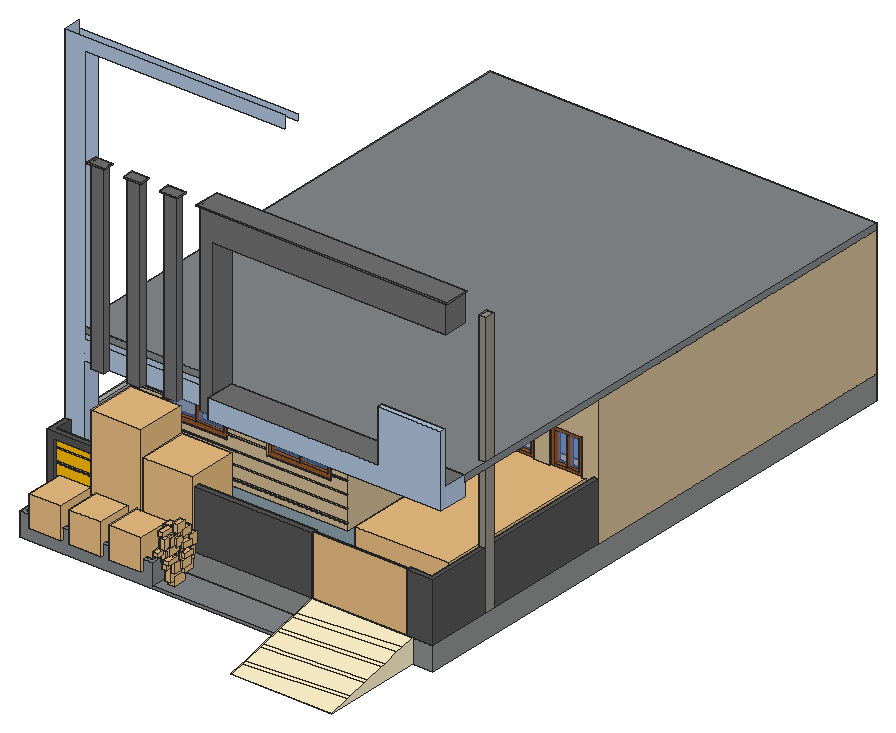
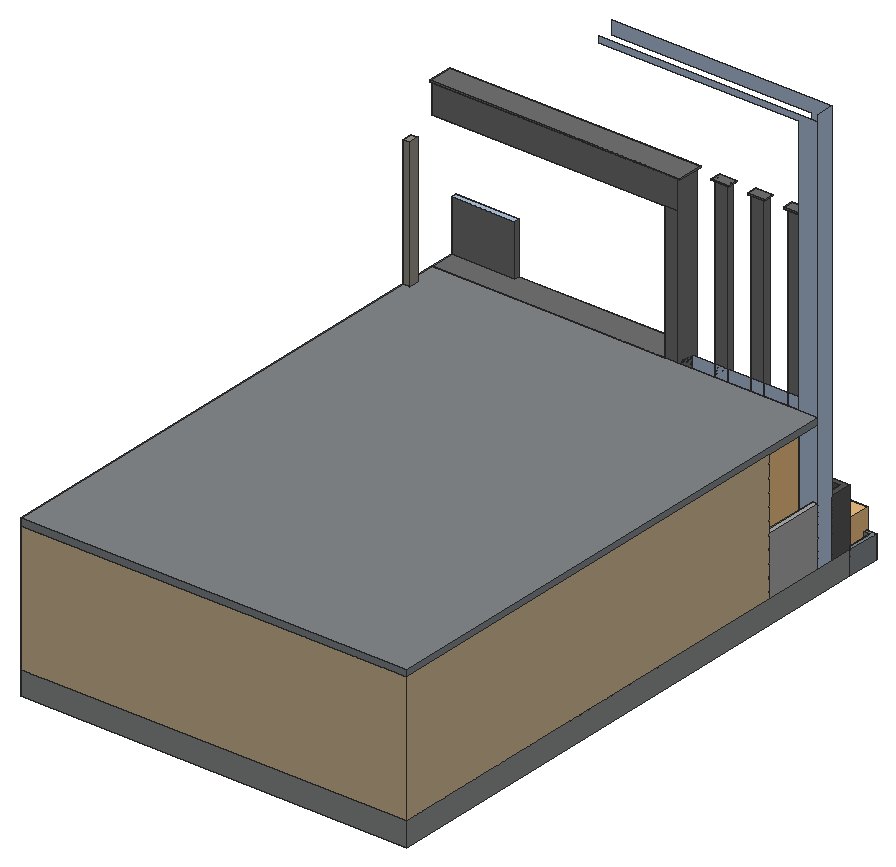
# SketchUp Ruby script. Lengths in inches.
U = 1.inch
M = Sketchup.active_model
def pt(a) = Geom::Point3d.new(a.map { |v| v * U })
def face(e, loops, mat)
  f = e.add_face(loops[0].map { |a| pt(a) })
  loops[1..].each { |l| e.add_face(l.map { |a| pt(a) }).erase! }
  f.material = f.back_material = mat if mat
  f
end
# faces: each face lists its corners as indices into pts; further lists are holes
def faces(e, pts, list, mat = nil) = list.each { |f| face(e, (f[0].is_a?(Array) ? f : [f]).map { |l| l.map { |i| pts[i] } }, mat) }
# xy, xz, yz: faces in a plane at the given z, y or x. An outline is a flat list of corners, or four numbers for a rectangle; further outlines are holes
def ring(l) = l.size == 4 ? [[l[0], l[1]], [l[2], l[1]], [l[2], l[3]], [l[0], l[3]]] : l.each_slice(2).to_a
def flat(e, list, mat, &to3) = list.each { |f| face(e, (f[0].is_a?(Array) ? f : [f]).map { |l| ring(l).map { |u, v| to3.(u, v) } }, mat) }
def xy(e, z, list, mat = nil) = flat(e, list, mat) { |x, y| [x, y, z] }
def xz(e, y, list, mat = nil) = flat(e, list, mat) { |x, z| [x, y, z] }
def yz(e, x, list, mat = nil) = flat(e, list, mat) { |y, z| [x, y, z] }
def lines(e, pts, list) = list.each { |a, b| e.add_line(pt(pts[a]), pt(pts[b])) }
# prism: a flat outline (further loops are holes) pulled along v
def prism(e, loops, v, mat = nil)
  f = face(e, loops, mat); d = Geom::Vector3d.new(v.map { |x| x * U })
  f.pushpull(f.normal.samedirection?(d) ? d.length : -d.length)
end
def box(e, o, s, mat = nil) = prism(e, [[o, [o[0] + s[0], o[1], o[2]], [o[0] + s[0], o[1] + s[1], o[2]], [o[0], o[1] + s[1], o[2]]]], [0, 0, s[2]], mat)
def at(x, y, z, deg = 0) = Geom::Transformation.translation(pt([x, y, z])) * Geom::Transformation.rotation(ORIGIN, Z_AXIS, deg.degrees)
def axes(o, x, y, z) = Geom::Transformation.new([*x, 0, *y, 0, *z, 0, *pt(o).to_a, 1])
def part(name) = M.definitions.add(name)
# library, detail: a bought-in or finely detailed component or shape, given as its bounding box
def library(name, o, s) = part(name).tap { |d| box(d.entities, o, s) }
def detail(e, o, s) = box(e.add_group.entities, o, s)
def put(e, d, t, mat = nil) = e.add_instance(d, t).tap { |i| i.material = mat if mat }
def group(e, t, mat = nil) = e.add_group.tap { |g| g.transformation = t; g.material = mat if mat }.entities
root = M.entities
M.materials.add("[0099_LightSteelBlue]").color = [176, 196, 222]
M.materials.add("[Blacktop Old 01]").color = [132, 136, 139]
M.materials.add("[Blacktop Old 02]").color = [143, 145, 145]
M.materials.add("[Color D01]").color = [255, 242, 204]
M.materials.add("[Color D04]").color = [255, 204, 50]
M.materials.add("[Color D05]").color = [255, 191, 0]
M.materials.add("[Color M03]").color = [170, 170, 170]
M.materials.add("[Color M05]").color = [114, 114, 114]
M.materials.add("[Color M06]").color = [86, 86, 86]
M.materials.add("[Formica Beige]").color = [211, 187, 149]
M.materials.add("[Formica Graystone]").color = [149, 146, 135]
M.materials.add("[Square Glass Tile 01]").color = [123, 142, 151]
M.materials.add("[Translucent Glass Blue]").color = [100, 149, 237]
M.materials["[Translucent Glass Blue]"].alpha = 0.5
M.materials.add("[Wood Cherry Original]").color = [152, 86, 42]
c1 = library("Group59\#1",[-32.98,33.92,22.15],[23.96,96.56,83.1])
c2 = library("Group60\#1",[-47.26,-81.53,115.8],[11.57,60.71,53.88])
c3 = library("Group61\#1",[17.15,84.19,16.4],[76.98,72.79,100.38])
c4 = library("Group62\#1",[-41.8,-20.16,82.85],[99.48,139.14,54.12])
c5 = library("Group63\#1",[-78.07,100.88,62.43],[61.26,81.43,86.37])
c6 = library("Group64\#1",[46.33,-12.9,51.95],[92.42,78.95,51.57])
c7 = library("Group65\#1",[-73.78,-20.03,120.09],[33.05,103.71,51.96])
c8 = library("Group66\#1",[-93.39,-19.9375,115.15],[70.74,15.37,89.07])
c9 = library("Group67\#1",[-160.6,-41.84,176.32],[92.55,73.84,45.89])
c10 = library("Group68\#1",[-72.58,-136.32,72.38],[80.41,85.97,95.72])
c11 = library("Group69\#1",[-107.89,47.83,91.71],[66.48,87.86,82.46])
c12 = library("Group70\#1",[-20.98,-42.53,-198.63],[46.69,46.24,172.61])
c13 = library("Group71\#1",[-0.8,-43.35,191.05],[81.04,80.57,74.82])
c14 = library("Group72\#1",[-44.16,-20.64,117.23],[64.94,35.73,104.26])
c15 = library("Group73\#2",[-85.2,-151.09,191.26],[83.6,108.34,38.47])
c16 = library("Group74\#1",[-43.32,-82.39,113.66],[8.74,67.58,95.91])
c17 = library("Group75\#1",[-19.52,-83.01,-122.96],[25.03,96.75,107.02])
c18 = library("Group76\#1",[-73.41,104.74,-36.57],[91.05,64.11,87.76])
c19 = library("Group77\#1",[6.72,-35.5625,-44.3],[97.86,50.43,71.28])
c20 = library("Group78\#1",[-46.16,95.67,-127.18],[89.22,60,98.58])
c21 = library("Group79\#1",[-73.36,-53.98,-265.87],[113.5,113.5,80.32])
c22 = library("Group80\#1",[-49.58,-31.64,-192.73],[34.2,35.75,335.89])
c23 = library("Group81\#1",[-33.25,31.15,20.5625],[19.21,100.94,38.88])
c24 = library("Group82\#1",[70.71,-26.24,-13.72],[94.01,86.31,40.81])
c25 = library("Group83\#1",[-78.76,-45.9375,-42.49],[89.36,13.07,73.45])
c26 = library("Group84\#1",[1.95,9.69,-124.66],[99.34,14.87,96.07])
c27 = library("Group85\#1",[5.34,-106.29,-47.41],[68.63,73.37,61.51])
c28 = library("Group86\#1",[4.23,10.03,-136.62],[40.98,41.87,51.36])
c29 = library("Group87\#1",[7.14,-44.59,-77.7],[48.84,15.98,59.8])
c30 = library("Group88\#1",[-32.7,-24.31,24.45],[55.13,61.32,79.5])
c31 = library("Group89\#1",[-77.24,-123.58,-46.56],[87.79,92.59,104.1])
c32 = library("Group90\#1",[-164.72,37.75,-20.84],[98.29,65.97,82.77])
c33 = library("Group91\#1",[-103.43,33.69,20.61],[71.41,32.36,40.62])
c34 = library("Group92\#1",[-125.68,-182.3125,23.5],[85.66,94.28,35.8])
c35 = library("Group93\#1",[5.2,-33.94,-67.23],[20.18,157.98,40.35])
c36 = library("Group94\#1",[2.39,9.02,-121.59],[42.15,71.34,93.56])
c37 = library("Group95\#1",[-55.3125,-129.29,-96.66],[79.37,72.9,68.93])
c38 = library("Group96\#1",[-140.7,-35.21,-77.44],[97.31,70.81,56.29])
c39 = library("Group97\#1",[-10.06,-56.42,72.68],[90.9,68.8,76.87])
c40 = library("Group98\#1",[12.8,58.29,-66.98],[80.58,78.21,79.14])
c41 = library("Group99\#1",[-35.4,-17.16,23.02],[118.23,50.83,58.94])
c42 = library("Group100\#1",[29.51,-171.04,-20.53],[91.11,101.22,39.04])
c43 = library("Group101\#1",[-97.95,11.13,-121.05],[102.09,51.91,53.69])
c44 = library("Group102\#1",[6.02,5.95,144.49],[89.45,87.47,55.68])
c45 = library("Group103\#1",[-45.73,-21.24,120.09],[87.14,68.72,79.33])
c46 = library("Group104\#1",[-32.38,-52.6,16.55],[60.96,98.07,53.51])
c47 = library("Group105\#1",[-69.28,-88.77,-223.3],[101.83,125.23,376.24])
c48 = library("Group106\#1",[-122.02,-42.04,23.03],[89.8,79.69,89.2])
c49 = library("Group107\#1",[-147.28,-98.05,24.68],[53.49,99.81,98.14])
c50 = library("Group108\#1",[38.95,-94,-129.36],[60.91,93.27,90.52])
c51 = library("Group109\#1",[-124.75,-75.19,-35.84],[77.11,72.51,79.94])
c52 = library("Group110\#1",[-78.58,0.56,-119.09],[84.31,12.02,77.58])
c53 = library("Group111\#1",[62.69,-31.6,-103.24],[86.45,84.15,71.79])
c54 = library("Group112\#1",[5.13,22.77,-174.65],[91.17,82.67,75.7])
c55 = library("Group113\#1",[-8.89,-115.37,23.85],[66.54,93.07,62.51])
c56 = library("Group114\#1",[-138.5625,33.88,-184.78],[81.4,51.14,109.21])
c57 = library("Group115\#1",[-39.22,1.8,-197.74],[25.16,42.04,242.32])
c58 = library("Group116\#1",[-16.77,0.31,-197.58],[31.04,19.97,97.43])
c59 = part("Group58\#1")
put(c59.entities,c1,at(0,0,0))
put(c59.entities,c2,at(0,0,0))
put(c59.entities,c3,at(0,0,0))
put(c59.entities,c4,at(0,0,0))
put(c59.entities,c5,at(0,0,0))
put(c59.entities,c6,at(0,0,0))
put(c59.entities,c7,at(0,0,0))
put(c59.entities,c8,at(0,0,0))
put(c59.entities,c9,at(0,0,0))
put(c59.entities,c10,at(0,0,0))
put(c59.entities,c11,at(0,0,0))
put(c59.entities,c12,at(0,0,0))
put(c59.entities,c13,at(0,0,0))
put(c59.entities,c14,at(0,0,0))
put(c59.entities,c15,at(0,0,0))
put(c59.entities,c16,at(0,0,0))
put(c59.entities,c17,at(0,0,0))
put(c59.entities,c18,at(0,0,0))
put(c59.entities,c19,at(0,0,0))
put(c59.entities,c20,at(0,0,0))
put(c59.entities,c21,at(0,0,0))
put(c59.entities,c22,at(0,0,0))
put(c59.entities,c23,at(0,0,0))
put(c59.entities,c24,at(0,0,0))
put(c59.entities,c25,at(0,0,0))
put(c59.entities,c26,at(0,0,0))
put(c59.entities,c27,at(0,0,0))
put(c59.entities,c28,at(0,0,0))
put(c59.entities,c29,at(0,0,0))
put(c59.entities,c30,at(0,0,0))
put(c59.entities,c31,at(0,0,0))
put(c59.entities,c32,at(0,0,0))
put(c59.entities,c33,at(0,0,0))
put(c59.entities,c34,at(0,0,0))
put(c59.entities,c35,at(0,0,0))
put(c59.entities,c36,at(0,0,0))
put(c59.entities,c37,at(0,0,0))
put(c59.entities,c38,at(0,0,0))
put(c59.entities,c39,at(0,0,0))
put(c59.entities,c40,at(0,0,0))
put(c59.entities,c41,at(0,0,0))
put(c59.entities,c42,at(0,0,0))
put(c59.entities,c43,at(0,0,0))
put(c59.entities,c44,at(0,0,0))
put(c59.entities,c45,at(0,0,0))
put(c59.entities,c46,at(0,0,0))
put(c59.entities,c47,at(0,0,0))
put(c59.entities,c48,at(0,0,0))
put(c59.entities,c49,at(0,0,0))
put(c59.entities,c50,at(0,0,0))
put(c59.entities,c51,at(0,0,0))
put(c59.entities,c52,at(0,0,0))
put(c59.entities,c53,at(0,0,0))
put(c59.entities,c54,at(0,0,0))
put(c59.entities,c55,at(0,0,0))
put(c59.entities,c56,at(0,0,0))
put(c59.entities,c57,at(0,0,0))
put(c59.entities,c58,at(0,0,0))
c60 = part("SimLab\#1")
put(c60.entities,c59,at(0,0,0))
c61 = library("mercy",[0,0.0625,0.17],[86.93,197.26,61.05])
c62 = library("SKT_Nearly Natural 5' Kentia Palm Silk Tree",[-23.18,-17.61,0],[47.48,43.95,59.125])
c63 = library("Untitled",[0,0,0],[36,4.39,84])
c64 = part("Group48\#1")
prism(c64.entities,[[[1382.99,-93.96,0],[1358.12,-93.96,0],[1358.12,-88.96,0],[1377.99,-88.96,0],[1377.99,98,0],[1382.99,98,0]]],[0,0,54.37])
c65 = part("Group50\#1")
box(c65.entities,[1024.5625,-57.52,0],[5,57.52,54.37])
c66 = part("Group51\#1")
xy(c66.entities,0,[[1024.5625,-93.96,1024.5625,-72.96,1029.5625,-72.96,1029.5625,-88.96,1270.5,-88.96,1270.5,-93.96,1136.9375,-93.96,1136.9375,-90.96,1030.5625,-90.96,1030.5625,-93.96]])
xy(c66.entities,3.55,[[1030.5625,-90.96,1136.9375,-89.96]])
xy(c66.entities,5.49,[[1030.5625,-90.96,1136.9375,-89.96]])
xy(c66.entities,15.37,[[1030.5625,-90.96,1136.9375,-89.96]])
xy(c66.entities,17.3,[[1030.5625,-90.96,1136.9375,-89.96]])
xy(c66.entities,27.18,[[1030.5625,-90.96,1136.9375,-89.96]])
xy(c66.entities,29.12,[[1030.5625,-90.96,1136.9375,-89.96]])
xy(c66.entities,38.99,[[1030.5625,-90.96,1136.9375,-89.96]])
xy(c66.entities,40.93,[[1030.5625,-90.96,1136.9375,-89.96]])
xy(c66.entities,48.37,[[1030.5625,-93.96,1136.9375,-90.96]])
xy(c66.entities,54.37,[[1024.5625,-93.96,1270.5,-93.96,1270.5,-88.96,1029.5625,-88.96,1029.5625,-72.96,1024.5625,-72.96]])
xz(c66.entities,-93.96,[[1024.5625,0,1030.5625,0,1030.5625,48.37,1136.9375,48.37,1136.9375,0,1270.5,0,1270.5,54.37,1024.5625,54.37]])
xz(c66.entities,-90.96,[[1030.5625,0,1136.9375,3.55]])
xz(c66.entities,-90.96,[[1030.5625,5.49,1136.9375,15.37],[1030.5625,17.3,1136.9375,27.18],[1030.5625,29.12,1136.9375,38.99],[1030.5625,40.93,1136.9375,48.37]],"[Color D05]")
xz(c66.entities,-89.96,[[1030.5625,3.55,1136.9375,5.49],[1030.5625,15.37,1136.9375,17.3]],"[Color D04]")
xz(c66.entities,-89.96,[[1030.5625,27.18,1136.9375,29.12],[1030.5625,38.99,1136.9375,40.93]],"[Color D05]")
xz(c66.entities,-88.96,[[1029.5625,0,1270.5,54.37]])
xz(c66.entities,-72.96,[[1024.5625,0,1029.5625,54.37]])
yz(c66.entities,1024.5625,[[-93.96,0,-72.96,54.37]])
yz(c66.entities,1029.5625,[[-88.96,0,-72.96,54.37]])
yz(c66.entities,1030.5625,[[-93.96,0,-90.96,48.37]])
yz(c66.entities,1136.9375,[[-93.96,0,-90.96,48.37]])
yz(c66.entities,1270.5,[[-93.96,0,-88.96,54.37]])
c67 = library("Untitled\#1",[131.66,19.68,0],[2.41,197.25,46.46])
c68 = part("Group4\#2")
xy(c68.entities,0,[[-26.0625,-20.0625,-0.59,20.0625],[0.59,-20.0625,26.0625,20.0625]])
c69 = part("Group3\#1")
prism(c69.entities,[[[-30,-24,0],[-30,24,0],[30,24,0],[30,-24,0]],[[26.0625,-20.0625,0],[26.0625,20.0625,0],[0.59,20.0625,0],[0.59,-20.0625,0]],[[-0.59,-20.0625,0],[-0.59,20.0625,0],[-26.0625,20.0625,0],[-26.0625,-20.0625,0]]],[0,0,5.875])
put(c69.entities,c68,at(0,0,2.9375),"[Translucent Glass Blue]")
c70 = part("Group6\#2")
xy(c70.entities,0,[[-26.0625,-20.0625,-0.59,20.0625],[0.59,-20.0625,26.0625,20.0625]])
c71 = part("Group5\#1")
prism(c71.entities,[[[-30,-24,0],[-30,24,0],[30,24,0],[30,-24,0]],[[0.59,20.0625,0],[0.59,-20.0625,0],[26.0625,-20.0625,0],[26.0625,20.0625,0]],[[-26.0625,-20.0625,0],[-0.59,-20.0625,0],[-0.59,20.0625,0],[-26.0625,20.0625,0]]],[0,0,5.875])
put(c71.entities,c70,at(0,0,2.9375),"[Translucent Glass Blue]")
c72 = part("Group8\#2")
xy(c72.entities,0,[[-11.0625,-14.0625,-0.59,14.0625],[0.59,-14.0625,11.0625,14.0625]])
c73 = part("Group7\#1")
prism(c73.entities,[[[-15,18,0],[15,18,0],[15,-18,0],[-15,-18,0]],[[11.0625,-14.0625,0],[11.0625,14.0625,0],[0.59,14.0625,0],[0.59,-14.0625,0]],[[-11.0625,-14.0625,0],[-0.59,-14.0625,0],[-0.59,14.0625,0],[-11.0625,14.0625,0]]],[0,0,5.875])
put(c73.entities,c72,at(0,0,2.9375),"[Translucent Glass Blue]")
c74 = part("Group10\#2")
xy(c74.entities,0,[[-10.5625,-14.0625,-0.59,14.0625],[0.59,-14.0625,10.5625,14.0625]])
c75 = part("Group9\#1")
prism(c75.entities,[[[14.5,18,0],[14.5,-18,0],[-14.5,-18,0],[-14.5,18,0]],[[0.59,-14.0625,0],[10.5625,-14.0625,0],[10.5625,14.0625,0],[0.59,14.0625,0]],[[-0.59,-14.0625,0],[-0.59,14.0625,0],[-10.5625,14.0625,0],[-10.5625,-14.0625,0]]],[0,0,5.875])
put(c75.entities,c74,at(0,0,2.9375),"[Translucent Glass Blue]")
xy(root,-21.875,[[245.9375,0,339.4375,93.625]],"[Color D01]")
xy(root,0,[[0,114.625,18,130.0625]],"[0099_LightSteelBlue]")
xy(root,108,[[18,114.625,130.05,130.0625]],"[0099_LightSteelBlue]")
xz(root,93.625,[[245.9375,-21.875,336.625,0],[336.625,-21.875,339.4375,0]])
xz(root,114.625,[[0,0,18,0,18,108,39.93,108,39.93,126,18,126,18,366,203.78,366,203.78,378,0,378],[39.93,108,130.05,126]],"[0099_LightSteelBlue]")
xz(root,130.0625,[[0,0,0,372,203.78,372,203.78,366,18,366,18,126,130.05,126,130.05,108,18,108,18,0]],"[0099_LightSteelBlue]")
yz(root,0,[[114.625,0,130.0625,378]],"[0099_LightSteelBlue]")
yz(root,18,[[114.625,0,130.0625,108]],"[0099_LightSteelBlue]")
yz(root,130.05,[[114.625,108,130.0625,126]],"[0099_LightSteelBlue]")
yz(root,245.9375,[[0,-21.875,12.76,-18.89,16.48,-18.03,32.95,-14.18,36.67,-13.31,52.92,-9.51,56.63,-8.64,70.5,-5.4,75.68,-4.19,93.625,0,93.625,-21.875]],"[Color D01]")
yz(root,339.4375,[[0,-21.875,93.625,-21.875,93.625,0,81.67,-2.79,75.68,-4.19,61.8,-7.43,58.09,-8.3,41.84,-12.1,38.13,-12.97,21.65,-16.82,17.94,-17.68]],"[Color D01]")
p = [[339.4375,0,-21.875],[339.4375,17.94,-17.68],[245.9375,12.76,-18.89],[245.9375,0,-21.875],[245.9375,16.48,-18.03],[339.4375,21.65,-16.82],
  [245.9375,32.95,-14.18],[339.4375,38.13,-12.97],[245.9375,36.67,-13.31],[339.4375,41.84,-12.1],[245.9375,52.92,-9.51],[339.4375,58.09,-8.3],
  [245.9375,56.63,-8.64],[339.4375,61.8,-7.43],[245.9375,70.5,-5.4],[339.4375,75.68,-4.19],[245.9375,75.68,-4.19],[339.4375,81.67,-2.79],
  [245.9375,93.625,0],[339.4375,93.625,0],[336.625,93.625,0],[31.9375,192.08,36],[31.9375,192.08,84],[91.9375,192.08,84],
  [91.9375,192.08,36],[128.47,192.08,36],[128.47,192.08,84],[188.47,192.08,84],[188.47,192.08,36],[269.16,290.08,48],
  [269.16,290.08,84],[298.16,290.08,84],[298.16,290.08,48],[312.74,290.08,48],[312.74,290.08,84],[342.74,290.08,84],
  [342.74,290.08,48],[245.9375,93.625,3.6875],[0,93.625,-21.875],[0,93.625,3.6875],[18,130.0625,114],[18,130.0625,108],
  [18,114.625,114]]
faces(root,p,[[0,1,2,3],[4,2,1,5],[6,4,5,7],[8,6,7,9],[10,8,9,11],[12,10,11,13],[14,12,13,15],[16,14,15,17],
  [18,16,17,19,20]],"[Color D01]")
lines(root,p,[[21,22],[22,23],[23,24],[24,21],[25,26],[26,27],[27,28],[28,25],[29,30],[30,31],[31,32],[32,29],
  [33,34],[34,35],[35,36],[36,33],[18,37],[38,39],[40,41],[42,40]])
g1 = group(root,at(0,187.58,-6),"[Square Glass Tile 01]")
xy(g1,-15.875,[[0,-93.96,358.43,420]],"[Blacktop Old 02]")
xy(g1,6,[[0,-93.96,358.43,420]])
xz(g1,-93.96,[[0,-15.875,358.43,6]],"[Blacktop Old 02]")
xz(g1,420,[[0,-15.875,358.43,6]],"[Blacktop Old 02]")
yz(g1,0,[[-93.96,-15.875,420,6]],"[Blacktop Old 02]")
yz(g1,358.43,[[-93.96,-15.875,420,6]],"[Blacktop Old 02]")
g2 = group(root,at(0,62.69,-21.875),"[Blacktop Old 01]")
xy(g2,0,[[0,0,245.9375,30.93]])
xy(g2,2.24,[[122.97,0,245.9375,30.93]])
xy(g2,11.3,[[3.35,3.35,119.62,27.59]])
xy(g2,21.875,[[[0,0,122.97,30.93],[3.35,3.35,119.62,27.59]]])
xz(g2,0,[[0,0,245.9375,0,245.9375,2.24,122.97,2.24,122.97,21.875,0,21.875]])
xz(g2,3.35,[[3.35,11.3,119.62,21.875]])
xz(g2,27.59,[[3.35,11.3,119.62,21.875]])
xz(g2,30.93,[[0,0,0,21.875,122.97,21.875,122.97,2.24,245.9375,2.24,245.9375,0]])
yz(g2,0,[[0,0,30.93,21.875]])
yz(g2,3.35,[[3.35,11.3,27.59,21.875]])
yz(g2,119.62,[[3.35,11.3,27.59,21.875]])
yz(g2,122.97,[[0,2.24,30.93,21.875]])
yz(g2,245.9375,[[0,0,30.93,2.24]])
put(root,c60,axes([135.92,74.36,8.74],[0.05714,0,0],[0,0.10569,0],[0,0,0.09711]))
put(root,c61,axes([259.47,126.22,-11.25],[1,0,0],[0,0.904,0],[0,0,1]))
put(root,c62,axes([23.92,79.35,-10.58],[0.62565,0,0],[0,1.04371,0],[0,0,0.48546]))
put(root,c62,axes([61.18,79.35,-10.58],[0.62565,0,0],[0,1.04371,0],[0,0,0.48546]))
put(root,c62,axes([98.45,79.35,-10.58],[0.62565,0,0],[0,1.04371,0],[0,0,0.48546]))
put(root,c62,axes([112.3,110.83,-1.16],[0.97,0,0],[0,1.04371,0],[0,0,1.0788]))
put(root,c62,axes([64.43,110.83,-1.16],[0.97,0,0],[0,1.04371,0],[0,0,1.45784]))
put(root,c63,at(217.22,287.67,0))
g3 = group(root,at(0,187.58,0),"[Formica Beige]")
xy(g3,0,[[0,0,0,420,358.43,420,358.43,98,253.22,98,253.22,107,349.43,107,349.43,411,9,411,9,9,194.78,9,194.78,107,217.22,107,217.22,98,203.78,98,203.78,0]])
xy(g3,5.19,[[0,0,203.78,1]])
xy(g3,7.12,[[0,0,203.78,1]])
xy(g3,17,[[0,0,203.78,1]])
xy(g3,18.94,[[0,0,203.78,1]])
xy(g3,28.81,[[0,0,203.78,1]])
xy(g3,30.75,[[0,0,203.78,1]])
xy(g3,36,[[31.9375,0,91.9375,9],[128.47,0,188.47,9]])
xy(g3,40.62,[[0,0,31.9375,1],[91.9375,0,128.47,1],[188.47,0,203.78,1]])
xy(g3,42.56,[[0,0,31.9375,1],[91.9375,0,128.47,1],[188.47,0,203.78,1]])
xy(g3,48,[[269.16,98,298.16,107],[312.74,98,342.74,107]])
xy(g3,52.44,[[0,0,31.9375,1],[91.9375,0,128.47,1],[188.47,0,203.78,1]])
xy(g3,54.37,[[0,0,31.9375,1],[91.9375,0,128.47,1],[188.47,0,203.78,1]])
xy(g3,64.25,[[0,0,31.9375,1],[91.9375,0,128.47,1],[188.47,0,203.78,1]])
xy(g3,66.19,[[0,0,31.9375,1],[91.9375,0,128.47,1],[188.47,0,203.78,1]])
xy(g3,76.06,[[0,0,31.9375,1],[91.9375,0,128.47,1],[188.47,0,203.78,1]])
xy(g3,78,[[0,0,31.9375,1],[91.9375,0,128.47,1],[188.47,0,203.78,1]])
xy(g3,84,[[31.9375,0,91.9375,9],[128.47,0,188.47,9],[217.22,98,253.22,107],[269.16,98,298.16,107],[312.74,98,342.74,107]])
xy(g3,87.87,[[0,0,203.78,1]])
xy(g3,89.81,[[0,0,203.78,1]])
xy(g3,99.69,[[0,0,203.78,1]])
xy(g3,101.62,[[0,0,203.78,1]])
xy(g3,111.5,[[0,0,203.78,1]])
xy(g3,113.44,[[0,0,203.78,1]])
xy(g3,120,[[[0,0,203.78,0,203.78,98,358.43,98,358.43,420,0,420],[9,9,9,411,349.43,411,349.43,107,194.78,107,194.78,9]]])
xz(g3,0,[[0,0,203.78,5.19],[0,7.12,203.78,17],[0,18.94,203.78,28.81],[0,30.75,203.78,30.75,203.78,40.62,188.47,40.62,188.47,36,128.47,36,128.47,40.62,91.9375,40.62,91.9375,36,31.9375,36,31.9375,40.62,0,40.62],[0,42.56,31.9375,52.44],
  [91.9375,42.56,128.47,52.44],[188.47,42.56,203.78,52.44],[0,54.37,31.9375,64.25],[91.9375,54.37,128.47,64.25],[188.47,54.37,203.78,64.25],
  [0,66.19,31.9375,76.06],[91.9375,66.19,128.47,76.06],[188.47,66.19,203.78,76.06],[0,78,31.9375,78,31.9375,84,91.9375,84,91.9375,78,128.47,78,128.47,84,188.47,84,188.47,78,203.78,78,203.78,87.87,0,87.87],[0,89.81,203.78,99.69],
  [0,101.62,203.78,111.5],[0,113.44,203.78,120]])
xz(g3,1,[[0,5.19,203.78,7.12],[0,17,203.78,18.94],[0,28.81,203.78,30.75],[0,40.62,31.9375,42.56],[91.9375,40.62,128.47,42.56],
  [188.47,40.62,203.78,42.56],[0,52.44,31.9375,54.37],[91.9375,52.44,128.47,54.37],[188.47,52.44,203.78,54.37],[0,64.25,31.9375,66.19],
  [91.9375,64.25,128.47,66.19],[188.47,64.25,203.78,66.19],[0,76.06,31.9375,78],[91.9375,76.06,128.47,78],[188.47,76.06,203.78,78],
  [0,87.87,203.78,89.81],[0,99.69,203.78,101.62],[0,111.5,203.78,113.44]])
xz(g3,9,[[[9,0,194.78,120],[31.9375,36,91.9375,84],[128.47,36,188.47,84]]])
xz(g3,98,[[[203.78,0,217.22,0,217.22,84,253.22,84,253.22,0,358.43,0,358.43,120,203.78,120],[312.74,48,342.74,84],[269.16,48,298.16,84]]])
xz(g3,107,[[[194.78,0,194.78,120,349.43,120,349.43,0,253.22,0,253.22,84,217.22,84,217.22,0],[312.74,48,342.74,84],[269.16,48,298.16,84]]])
xz(g3,411,[[9,0,349.43,120]])
xz(g3,420,[[0,0,358.43,120]])
yz(g3,0,[[0,0,0,5.19,1,5.19,1,7.12,0,7.12,0,17,1,17,1,18.94,0,18.94,0,28.81,1,28.81,1,30.75,0,30.75,0,40.62,1,40.62,1,42.56,0,42.56,0,52.44,1,52.44,1,54.37,0,54.37,0,64.25,1,64.25,1,66.19,0,66.19,0,76.06,1,76.06,1,78,0,78,0,87.87,1,87.87,1,89.81,0,89.81,0,99.69,1,99.69,1,101.62,0,101.62,0,111.5,1,111.5,1,113.44,0,113.44,0,120,420,120,420,0],[0,5.19,1,7.12],[0,17,1,18.94],[0,28.81,1,30.75],[0,40.62,1,42.56]])
yz(g3,9,[[9,0,411,120]])
yz(g3,31.9375,[[0,36,9,36,9,84,0,84,0,78,1,78,1,76.06,0,76.06,0,66.19,1,66.19,1,64.25,0,64.25,0,54.37,1,54.37,1,52.44,0,52.44,0,42.56,1,42.56,1,40.62,0,40.62],[0,52.44,1,54.37],[0,64.25,1,66.19],[0,76.06,1,78]])
yz(g3,91.9375,[[0,36,0,40.62,1,40.62,1,42.56,0,42.56,0,52.44,1,52.44,1,54.37,0,54.37,0,64.25,1,64.25,1,66.19,0,66.19,0,76.06,1,76.06,1,78,0,78,0,84,9,84,9,36],[0,40.62,1,42.56],[0,52.44,1,54.37],[0,64.25,1,66.19],[0,76.06,1,78]])
yz(g3,128.47,[[0,36,9,36,9,84,0,84,0,78,1,78,1,76.06,0,76.06,0,66.19,1,66.19,1,64.25,0,64.25,0,54.37,1,54.37,1,52.44,0,52.44,0,42.56,1,42.56,1,40.62,0,40.62],[0,40.62,1,42.56],[0,52.44,1,54.37],[0,64.25,1,66.19],[0,76.06,1,78]])
yz(g3,188.47,[[0,36,0,40.62,1,40.62,1,42.56,0,42.56,0,52.44,1,52.44,1,54.37,0,54.37,0,64.25,1,64.25,1,66.19,0,66.19,0,76.06,1,76.06,1,78,0,78,0,84,9,84,9,36],[0,40.62,1,42.56],[0,52.44,1,54.37],[0,64.25,1,66.19],[0,76.06,1,78]])
yz(g3,194.78,[[9,0,107,120]])
yz(g3,203.78,[[0,0,98,0,98,120,0,120,0,113.44,1,113.44,1,111.5,0,111.5,0,101.62,1,101.62,1,99.69,0,99.69,0,89.81,1,89.81,1,87.87,0,87.87,0,78,1,78,1,76.06,0,76.06,0,66.19,1,66.19,1,64.25,0,64.25,0,54.37,1,54.37,1,52.44,0,52.44,0,42.56,1,42.56,1,40.62,0,40.62,0,30.75,1,30.75,1,28.81,0,28.81,0,18.94,1,18.94,1,17,0,17,0,7.12,1,7.12,1,5.19,0,5.19]])
yz(g3,217.22,[[98,0,107,84]])
yz(g3,253.22,[[98,0,107,84]])
yz(g3,269.16,[[98,48,107,84]])
yz(g3,298.16,[[98,48,107,84]])
yz(g3,312.74,[[98,48,107,84]])
yz(g3,342.74,[[98,48,107,84]])
yz(g3,349.43,[[107,0,411,120]])
yz(g3,358.43,[[98,0,420,120]])
put(root,c64,at(-1024.5625,187.58,0),"[Color M06]")
g4 = group(root,at(352.43,154.46,126),"[Formica Graystone]")
box(g4,[0,0,-126],[6,9,246])
put(root,c65,at(-1024.5625,187.58,0),"[Color M03]")
put(root,c66,at(-1024.5625,187.58,0),"[Color M06]")
put(root,c67,axes([342.3,-37.16,0],[0,1,0],[-0.4442,0,0],[0,0,1.1704]))
put(root,c69,axes([61.9375,195.02,60],[1,0,0],[0,0,1],[0,-1,0]),"[Wood Cherry Original]")
put(root,c71,axes([158.47,195.02,60],[1,0,0],[0,0,1],[0,-1,0]),"[Wood Cherry Original]")
put(root,c73,axes([327.74,293.02,66],[1,0,0],[0,0,1],[0,-1,0]),"[Wood Cherry Original]")
put(root,c75,axes([283.66,293.02,66],[1,0,0],[0,0,1],[0,-1,0]),"[Wood Cherry Original]")
g5 = group(root,at(28.96,114.625,108),"[Color M05]")
xy(g5,0,[[0,-6,12,0]])
xy(g5,170.6875,[[-2,-8,14,-6],[-2,-6,0,2],[0,-6,12,0],[12,-6,14,2],[0,0,12,2]])
xy(g5,171.75,[[-2,-8,14,2]])
xz(g5,-8,[[-2,170.6875,14,171.75]])
xz(g5,-6,[[0,0,12,170.6875]])
xz(g5,0,[[0,0,12,170.6875]])
xz(g5,2,[[-2,170.6875,14,171.75]])
yz(g5,-2,[[-8,170.6875,2,171.75]])
yz(g5,0,[[-6,0,0,170.6875]])
yz(g5,12,[[-6,0,0,170.6875]])
yz(g5,14,[[-8,170.6875,2,171.75]])
g6 = group(root,at(130.05,130.0625,234),"[Color M05]")
xy(g6,-126,[[12,-27.4375,228.375,0],[0,-21.4375,12,0]])
xy(g6,-108,[[12,-27.4375,169.29,-27.4375,169.29,-22.4375,228.375,-22.4375,228.375,0,12,0]])
xy(g6,-60,[[169.29,-27.4375,228.375,-22.4375]],"[0099_LightSteelBlue]")
xy(g6,18,[[12,-21.4375,228.375,0]])
xy(g6,44.6875,[[-2,-23.4375,230.375,-21.4375],[-2,-21.4375,0,0],[0,-21.4375,228.375,0],[228.375,-21.4375,230.375,0]])
xy(g6,45.75,[[-2,-23.4375,230.375,0]])
xz(g6,-27.4375,[[12,-126,228.375,-126,228.375,-60,169.29,-60,169.29,-108,12,-108]],"[0099_LightSteelBlue]")
xz(g6,-23.4375,[[-2,44.6875,230.375,45.75]])
xz(g6,-22.4375,[[169.29,-108,228.375,-60]])
xz(g6,-21.4375,[[0,-126,12,-126,12,18,228.375,18,228.375,44.6875,0,44.6875]])
xz(g6,0,[[0,-126,12,18],[12,-126,228.375,-108],[0,18,228.375,44.6875],[-2,44.6875,230.375,45.75]])
yz(g6,-2,[[-23.4375,44.6875,0,45.75]])
yz(g6,0,[[-21.4375,-126,0,44.6875]])
yz(g6,12,[[-27.4375,-126,-21.4375,-108],[-21.4375,-126,0,-108],[-21.4375,-108,0,18]])
yz(g6,169.29,[[-27.4375,-108,-22.4375,-60]])
yz(g6,228.375,[[-21.4375,18,0,44.6875]])
yz(g6,228.375,[[-27.4375,-126,0,-126,0,-108,-22.4375,-108,-22.4375,-60,-27.4375,-60]],"[0099_LightSteelBlue]")
yz(g6,230.375,[[-23.4375,44.6875,0,45.75]])
g7 = group(root,at(96.09,114.625,108),"[Color M05]")
xy(g7,0,[[0,-6,12,0]])
xy(g7,170.6875,[[-2,-8,14,-6],[-2,-6,0,2],[0,-6,12,0],[12,-6,14,2],[0,0,12,2]])
xy(g7,171.75,[[-2,-8,14,2]])
xz(g7,-8,[[-2,170.6875,14,171.75]])
xz(g7,-6,[[0,0,12,170.6875]])
xz(g7,0,[[0,0,12,170.6875]])
xz(g7,2,[[-2,170.6875,14,171.75]])
yz(g7,-2,[[-8,170.6875,2,171.75]])
yz(g7,0,[[-6,0,0,170.6875]])
yz(g7,12,[[-6,0,0,170.6875]])
yz(g7,14,[[-8,170.6875,2,171.75]])
g8 = group(root,at(62.53,114.625,108),"[Color M05]")
xy(g8,0,[[0,-6,12,0]])
xy(g8,170.6875,[[-2,-8,0,2],[0,-8,14,-6],[0,-6,12,0],[12,-6,14,2],[0,0,12,2]])
xy(g8,171.75,[[-2,-8,14,2]])
xz(g8,-8,[[-2,170.6875,14,171.75]])
xz(g8,-6,[[0,0,12,170.6875]])
xz(g8,0,[[0,0,12,170.6875]])
xz(g8,2,[[-2,170.6875,14,171.75]])
yz(g8,-2,[[-8,170.6875,2,171.75]])
yz(g8,0,[[-6,0,0,170.6875]])
yz(g8,12,[[-6,0,0,170.6875]])
yz(g8,14,[[-8,170.6875,2,171.75]])
g9 = group(root,at(0,187.58,120),"[Blacktop Old 01]")
box(g9,[0,-57.52,0],[358.43,477.52,6])
